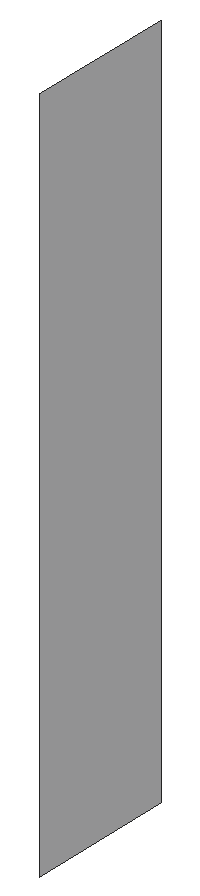
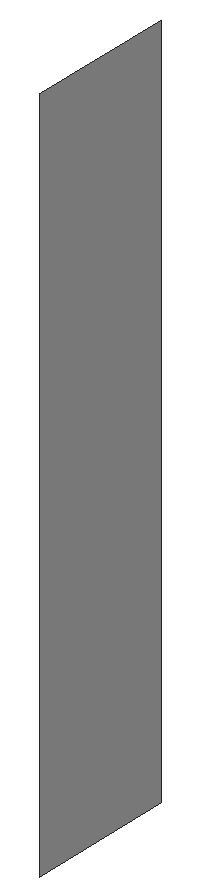
# SketchUp Ruby script. Lengths in inches.
U = 1.inch
M = Sketchup.active_model
def pt(a) = Geom::Point3d.new(a.map { |v| v * U })
def face(e, loops, mat)
  f = e.add_face(loops[0].map { |a| pt(a) })
  loops[1..].each { |l| e.add_face(l.map { |a| pt(a) }).erase! }
  f.material = f.back_material = mat if mat
  f
end
# faces: each face lists its corners as indices into pts; further lists are holes
def faces(e, pts, list, mat = nil) = list.each { |f| face(e, (f[0].is_a?(Array) ? f : [f]).map { |l| l.map { |i| pts[i] } }, mat) }
# xy, xz, yz: faces in a plane at the given z, y or x. An outline is a flat list of corners, or four numbers for a rectangle; further outlines are holes
def ring(l) = l.size == 4 ? [[l[0], l[1]], [l[2], l[1]], [l[2], l[3]], [l[0], l[3]]] : l.each_slice(2).to_a
def flat(e, list, mat, &to3) = list.each { |f| face(e, (f[0].is_a?(Array) ? f : [f]).map { |l| ring(l).map { |u, v| to3.(u, v) } }, mat) }
def xy(e, z, list, mat = nil) = flat(e, list, mat) { |x, y| [x, y, z] }
def xz(e, y, list, mat = nil) = flat(e, list, mat) { |x, z| [x, y, z] }
def yz(e, x, list, mat = nil) = flat(e, list, mat) { |y, z| [x, y, z] }
def lines(e, pts, list) = list.each { |a, b| e.add_line(pt(pts[a]), pt(pts[b])) }
# prism: a flat outline (further loops are holes) pulled along v
def prism(e, loops, v, mat = nil)
  f = face(e, loops, mat); d = Geom::Vector3d.new(v.map { |x| x * U })
  f.pushpull(f.normal.samedirection?(d) ? d.length : -d.length)
end
def box(e, o, s, mat = nil) = prism(e, [[o, [o[0] + s[0], o[1], o[2]], [o[0] + s[0], o[1] + s[1], o[2]], [o[0], o[1] + s[1], o[2]]]], [0, 0, s[2]], mat)
def at(x, y, z, deg = 0) = Geom::Transformation.translation(pt([x, y, z])) * Geom::Transformation.rotation(ORIGIN, Z_AXIS, deg.degrees)
def axes(o, x, y, z) = Geom::Transformation.new([*x, 0, *y, 0, *z, 0, *pt(o).to_a, 1])
def part(name) = M.definitions.add(name)
# library, detail: a bought-in or finely detailed component or shape, given as its bounding box
def library(name, o, s) = part(name).tap { |d| box(d.entities, o, s) }
def detail(e, o, s) = box(e.add_group.entities, o, s)
def put(e, d, t, mat = nil) = e.add_instance(d, t).tap { |i| i.material = mat if mat }
def group(e, t, mat = nil) = e.add_group.tap { |g| g.transformation = t; g.material = mat if mat }.entities
root = M.entities
M.materials.add("[Fencing Metal Straight]").color = [194, 195, 196]
yz(root,113.3,[[0,17.625,21.02,115.1875]],"[Fencing Metal Straight]")
